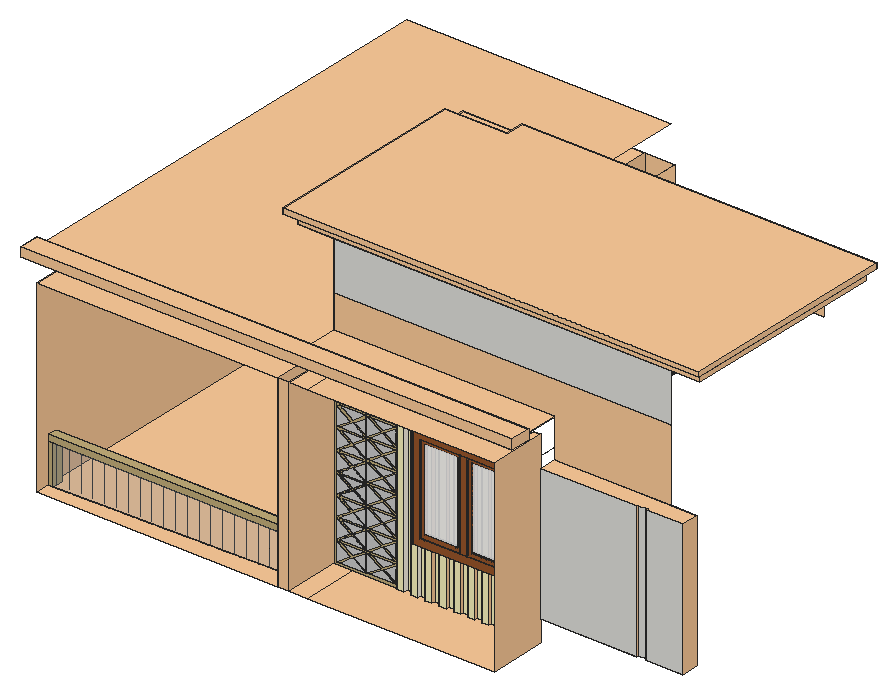
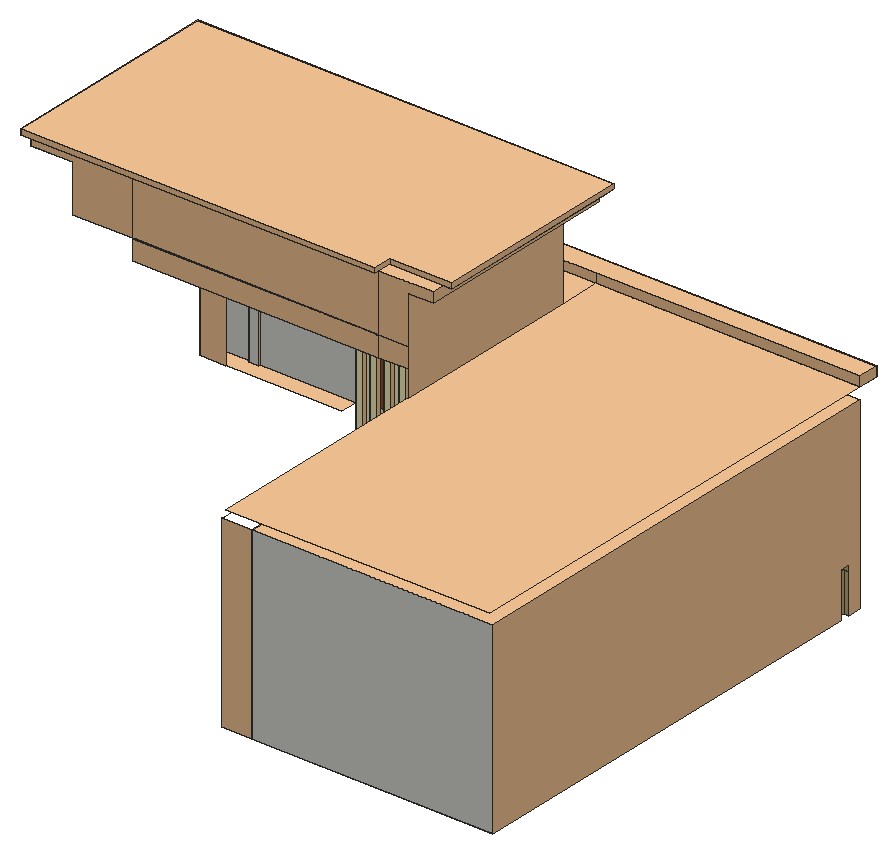
# SketchUp Ruby script. Lengths in inches.
U = 1.inch
M = Sketchup.active_model
def pt(a) = Geom::Point3d.new(a.map { |v| v * U })
def face(e, loops, mat)
  f = e.add_face(loops[0].map { |a| pt(a) })
  loops[1..].each { |l| e.add_face(l.map { |a| pt(a) }).erase! }
  f.material = f.back_material = mat if mat
  f
end
# faces: each face lists its corners as indices into pts; further lists are holes
def faces(e, pts, list, mat = nil) = list.each { |f| face(e, (f[0].is_a?(Array) ? f : [f]).map { |l| l.map { |i| pts[i] } }, mat) }
# xy, xz, yz: faces in a plane at the given z, y or x. An outline is a flat list of corners, or four numbers for a rectangle; further outlines are holes
def ring(l) = l.size == 4 ? [[l[0], l[1]], [l[2], l[1]], [l[2], l[3]], [l[0], l[3]]] : l.each_slice(2).to_a
def flat(e, list, mat, &to3) = list.each { |f| face(e, (f[0].is_a?(Array) ? f : [f]).map { |l| ring(l).map { |u, v| to3.(u, v) } }, mat) }
def xy(e, z, list, mat = nil) = flat(e, list, mat) { |x, y| [x, y, z] }
def xz(e, y, list, mat = nil) = flat(e, list, mat) { |x, z| [x, y, z] }
def yz(e, x, list, mat = nil) = flat(e, list, mat) { |y, z| [x, y, z] }
def lines(e, pts, list) = list.each { |a, b| e.add_line(pt(pts[a]), pt(pts[b])) }
# prism: a flat outline (further loops are holes) pulled along v
def prism(e, loops, v, mat = nil)
  f = face(e, loops, mat); d = Geom::Vector3d.new(v.map { |x| x * U })
  f.pushpull(f.normal.samedirection?(d) ? d.length : -d.length)
end
def box(e, o, s, mat = nil) = prism(e, [[o, [o[0] + s[0], o[1], o[2]], [o[0] + s[0], o[1] + s[1], o[2]], [o[0], o[1] + s[1], o[2]]]], [0, 0, s[2]], mat)
def at(x, y, z, deg = 0) = Geom::Transformation.translation(pt([x, y, z])) * Geom::Transformation.rotation(ORIGIN, Z_AXIS, deg.degrees)
def axes(o, x, y, z) = Geom::Transformation.new([*x, 0, *y, 0, *z, 0, *pt(o).to_a, 1])
def part(name) = M.definitions.add(name)
# library, detail: a bought-in or finely detailed component or shape, given as its bounding box
def library(name, o, s) = part(name).tap { |d| box(d.entities, o, s) }
def detail(e, o, s) = box(e.add_group.entities, o, s)
def put(e, d, t, mat = nil) = e.add_instance(d, t).tap { |i| i.material = mat if mat }
def group(e, t, mat = nil) = e.add_group.tap { |g| g.transformation = t; g.material = mat if mat }.entities
root = M.entities
M.materials.add("C02_Golden_Beige").color = [255, 205, 155]
M.materials.add("D02_Buttercup_Glow").color = [255, 248, 232]
M.materials.add("Glass_Basic_1").color = [161, 173, 186]
M.materials["Glass_Basic_1"].alpha = 0.25
M.materials.add("Metal_10_1K").color = [196, 175, 123]
M.materials.add("Metal_Perforated_03_1K").color = [205, 205, 205]
M.materials.add("Wood_Floor_01_1K").color = [255, 248, 193]
M.materials.add("[Translucent Glass Sky Reflection]").color = [253, 253, 253]
M.materials["[Translucent Glass Sky Reflection]"].alpha = 0.9
M.materials.add("[Wood Cherry Original]").color = [152, 86, 42]
c1 = library("Windows_Triple-Wood-Casement-Window-51inx36in",[0,0,-2.19],[51,41,3.19])
c2 = part("WINDOW")
g1 = group(c2.entities,at(4,1,4),"[Translucent Glass Sky Reflection]")
xy(g1,0,[[0,0,22,2]])
xy(g1,2,[[2,0,20,0.68],[2,0.68,20,2]],"[Wood Cherry Original]")
xy(g1,46,[[2,0,20,0.68],[2,0.68,20,2]],"[Wood Cherry Original]")
xy(g1,48,[[0,0,22,2]])
xz(g1,0,[[[0,0,22,48],[2,2,20,46]]],"[Wood Cherry Original]")
xz(g1,0.68,[[2,2,20,46]])
xz(g1,2,[[[0,0,22,48],[2,2,20,46]]],"[Wood Cherry Original]")
yz(g1,0,[[0,0,2,48]])
yz(g1,2,[[0,2,0.68,46],[0.68,2,2,46]],"[Wood Cherry Original]")
yz(g1,20,[[0,2,0.68,46],[0.68,2,2,46]],"[Wood Cherry Original]")
yz(g1,22,[[0,0,2,48]])
g2 = group(c2.entities,at(30,1,4),"[Translucent Glass Sky Reflection]")
xy(g2,0,[[0,0,22,2]])
xy(g2,2,[[2,0,20,0.68],[2,0.68,20,2]],"[Wood Cherry Original]")
xy(g2,46,[[2,0,20,0.68],[2,0.68,20,2]],"[Wood Cherry Original]")
xy(g2,48,[[0,0,22,2]])
xz(g2,0,[[[0,0,22,48],[2,2,20,46]]],"[Wood Cherry Original]")
xz(g2,0.68,[[2,2,20,46]])
xz(g2,2,[[[0,0,22,48],[2,2,20,46]]],"[Wood Cherry Original]")
yz(g2,0,[[0,0,2,48]])
yz(g2,2,[[0,2,0.68,46],[0.68,2,2,46]],"[Wood Cherry Original]")
yz(g2,20,[[0,2,0.68,46],[0.68,2,2,46]],"[Wood Cherry Original]")
yz(g2,22,[[0,0,2,48]])
g3 = group(c2.entities,at(0,0,0),"[Wood Cherry Original]")
xy(g3,0,[[0,0,56,4]])
xy(g3,4,[[4,0,26,4],[26,0,30,4],[30,0,52,4]])
xy(g3,52,[[4,0,26,4],[26,0,30,4],[30,0,52,4]])
xy(g3,56,[[0,0,56,4]])
xz(g3,0,[[[0,0,56,56],[4,4,52,52]],[26,4,30,52]])
xz(g3,4,[[[0,0,56,56],[4,4,52,52]],[26,4,30,52]])
yz(g3,0,[[0,0,4,56]])
yz(g3,4,[[0,4,4,52]])
yz(g3,26,[[0,4,4,52]])
yz(g3,30,[[0,4,4,52]])
yz(g3,52,[[0,4,4,52]])
yz(g3,56,[[0,0,4,56]])
xy(root,164.341,[[453.588,382.491,622.52,382.491,622.52,396.249,457.114,392.701,453.588,392.701],[630.52,382.491,643.626,422.102],[643.626,382.491,774.437,382.491,774.437,422.996,769.485,422.996,769.485,420.858,764.533,420.858,764.533,422.996,759.581,422.996,759.581,420.858,754.629,420.858,754.629,422.996,749.677,422.996,749.677,420.858,744.725,420.858,744.725,422.996,739.773,422.996,739.773,420.858,734.821,420.858,734.821,422.996,729.869,422.996,729.869,420.858,724.917,420.858,724.917,422.996,719.965,422.996,719.965,420.858,715.013,420.858,715.013,422.996,710.061,422.996,710.061,420.858,705.109,420.858,705.109,422.996,700.157,422.996,700.157,420.858,695.205,420.858,695.205,422.996,690.253,422.996,690.253,420.858,685.301,420.858,685.301,424.064,680.349,424.064,680.349,420.858,675.397,420.858,675.397,422.102,643.626,422.102],[457.114,392.701,622.52,396.249,622.52,703.99,453.588,703.99,453.588,399.796,457.114,399.796]],"C02_Golden_Beige")
xy(root,189.298,[[784.979,409.652,784.979,422.102,884.742,422.102,884.742,409.652,859.112,409.652,859.112,410.875,852.431,410.875,852.431,409.652]],"C02_Golden_Beige")
xy(root,191.701,[[457.114,392.701,457.114,399.796,622.52,399.796,622.52,396.249],[457.114,392.701,622.52,396.249,622.52,392.701]],"Metal_10_1K")
xy(root,196.087,[[453.588,392.701,622.52,399.796]],"Metal_10_1K")
xy(root,283.565,[[784.979,409.652,852.431,409.652,852.431,410.875,859.112,410.875,859.112,409.652,884.742,409.652,884.742,422.102,784.979,422.102]],"C02_Golden_Beige")
xy(root,295.512,[[[453.588,382.491,622.52,703.99],[484.212,419.811,491.847,605.683],[563.338,419.811,570.973,605.683]],[630.52,382.491,643.626,422.102],[643.626,382.491,643.626,422.102,675.397,422.102,675.397,420.858,680.349,420.858,680.349,424.064,685.301,424.064,685.301,420.858,690.253,420.858,690.253,422.996,695.205,422.996,695.205,420.858,700.157,420.858,700.157,422.996,705.109,422.996,705.109,420.858,710.061,420.858,710.061,422.996,715.013,422.996,715.013,420.858,719.965,420.858,719.965,422.996,724.917,422.996,724.917,420.858,729.869,420.858,729.869,422.996,734.821,422.996,734.821,420.858,739.773,420.858,739.773,422.996,744.725,422.996,744.725,420.858,749.677,420.858,749.677,422.996,754.629,422.996,754.629,420.858,759.581,420.858,759.581,422.996,764.533,422.996,764.533,420.858,769.485,420.858,769.485,422.996,774.437,422.996,774.437,382.491]],"C02_Golden_Beige")
xy(root,296.545,[[484.212,419.811,491.847,605.683]],"C02_Golden_Beige")
xy(root,298.092,[[563.338,419.811,570.973,605.683]],"C02_Golden_Beige")
xy(root,311.036,[[445.588,378.263,790.029,382.491],[445.588,382.491,784.979,392.701],[784.979,382.491,790.029,392.701],[445.588,392.701,630.52,716.631],[630.52,392.701,784.979,422.102]],"C02_Golden_Beige")
xy(root,317.496,[[445.588,378.263,790.029,392.701]],"C02_Golden_Beige")
xy(root,376.07,[[613.616,411.241,630.52,556.188],[630.52,411.241,895.57,422.102],[866.193,422.102,895.57,556.188]],"C02_Golden_Beige")
xy(root,383.319,[[608.019,405.157,899.824,411.241],[608.019,411.241,613.616,547.254],[895.57,411.241,899.824,560.283],[613.616,547.254,651.626,556.188],[651.626,556.188,823.98,560.283],
  [823.98,556.188,895.57,560.283]],"C02_Golden_Beige")
xy(root,386.847,[[608.019,405.157,899.824,405.157,899.824,560.283,651.626,560.283,651.626,547.254,608.019,547.254]],"C02_Golden_Beige")
xz(root,378.263,[[445.588,311.036,790.029,317.496]],"C02_Golden_Beige")
xz(root,382.491,[[622.52,164.341,630.52,295.512]],"C02_Golden_Beige")
xz(root,392.701,[[445.588,311.036,630.52,317.496],[630.52,311.036,790.029,317.496]],"C02_Golden_Beige")
xz(root,392.701,[[453.588,164.341,457.114,191.701],[453.588,191.701,622.52,196.087]],"Metal_10_1K")
xz(root,399.796,[[453.588,164.341,453.588,196.087,622.52,196.087,622.52,191.701,457.114,191.701,457.114,164.341]],"C02_Golden_Beige")
xz(root,405.157,[[608.019,383.319,899.824,386.847]],"C02_Golden_Beige")
xz(root,409.652,[[784.979,189.298,852.431,283.565],[859.112,189.298,884.742,283.565]])
xz(root,410.875,[[852.431,189.298,859.112,283.565]])
xz(root,411.241,[[613.616,376.07,895.57,383.319]],"C02_Golden_Beige")
xz(root,419.811,[[484.212,295.512,491.847,296.545],[563.338,295.512,570.973,298.092]],"C02_Golden_Beige")
xz(root,420.858,[[675.397,164.341,680.349,295.512],[685.301,164.341,690.253,295.512],[695.205,164.341,700.157,295.512],[705.109,164.341,710.061,295.512],[715.013,164.341,719.965,295.512],
  [724.917,164.341,729.869,295.512],[734.821,164.341,739.773,295.512],[744.725,164.341,749.677,295.512],[754.629,164.341,759.581,295.512],[764.533,164.341,769.485,295.512]],"Wood_Floor_01_1K")
xz(root,422.102,[[652.387,166.24,652.391,179.253],[652.387,180.373,652.387,180.535,652.139,180.535],[652.387,265.24,652.391,266.349],[652.387,266.349,652.391,279.363],[632.419,279.363,652.387,279.49],
  [630.52,334.01,866.193,376.07]])
xz(root,422.102,[[866.193,189.298,884.742,283.565],[784.979,283.565,866.193,283.565,866.193,334.01,630.52,334.01,630.52,311.036,784.979,311.036]],"C02_Golden_Beige")
xz(root,422.102,[[[630.52,164.341,675.397,295.512],[632.419,166.24,673.498,293.613]],[632.419,166.24,634.334,166.24,643.309,172.156,652.387,166.24,652.387,167.401,644.224,172.76,652.387,178.14,652.387,179.253,643.327,173.349,634.334,179.253,632.419,179.253,642.403,172.747],[[632.419,166.24,634.334,166.24,643.309,172.156,652.387,166.24,652.387,167.401,644.224,172.76,652.387,178.14,652.387,181.534,644.224,186.893,652.387,192.274,652.387,195.667,644.224,201.026,652.387,206.407,652.387,209.8,644.224,215.159,652.387,220.54,652.387,223.934,644.224,229.293,652.387,234.673,652.387,238.067,644.224,243.426,652.387,248.807,652.387,251.201,652.139,251.201,652.387,251.039,632.419,251.039,632.419,249.92,642.403,243.413,632.419,236.906,634.334,236.906,634.579,237.068,643.309,242.822,652.387,236.906,632.419,236.906,632.419,235.786,642.403,229.279,632.419,222.773,634.334,222.773,643.309,228.689,652.387,222.773,632.419,222.773,632.419,221.653,642.403,215.146,632.419,208.639,634.334,208.639,643.309,214.556,652.387,208.639,632.419,208.639,632.419,207.52,642.403,201.013,632.419,194.506,634.334,194.506,643.309,200.423,652.387,194.506,632.419,194.506,632.419,193.387,642.403,186.88,632.419,180.373,634.334,180.373,643.309,186.289,652.139,180.535,652.387,180.373,632.419,180.373,632.419,179.253,642.403,172.747],[643.327,173.349,634.334,179.253,652.387,179.253],[643.327,187.482,634.334,193.387,652.387,193.387],[643.327,201.615,634.334,207.52,652.387,207.52],[643.327,215.749,634.334,221.653,652.387,221.653],[643.327,229.882,634.334,235.786,652.387,235.786],[643.327,244.015,634.334,249.92,652.387,249.92]],[652.391,166.24,653.525,166.24,653.525,279.49,652.387,279.49,652.387,279.363,652.391,279.363,652.391,265.24,652.387,265.24,652.387,179.253,652.391,179.253],[653.525,166.24,655.44,166.24,664.415,172.156,673.493,166.24,673.493,167.401,665.331,172.76,673.493,178.14,673.493,179.253,664.434,173.349,655.44,179.253,653.525,179.253,663.509,172.747],
  [653.525,179.253,673.498,180.535],[632.419,180.373,634.334,180.373,643.309,186.289,652.139,180.535,652.387,180.535,652.387,181.534,644.224,186.893,652.387,192.274,652.387,193.387,643.327,187.482,634.334,193.387,632.419,193.387,642.403,186.88],[653.525,180.535,655.44,180.535,664.415,186.451,673.493,180.535,673.493,181.696,665.331,187.055,673.493,192.435,673.493,193.548,664.434,187.644,655.44,193.548,653.525,193.548,663.509,187.042],[653.525,193.548,673.498,194.83],[632.419,194.506,634.334,194.506,643.309,200.423,652.387,194.506,652.387,195.667,644.224,201.026,652.387,206.407,652.387,207.52,643.327,201.615,634.334,207.52,632.419,207.52,642.403,201.013],
  [653.525,194.83,655.44,194.83,664.415,200.746,673.493,194.83,673.493,195.991,665.331,201.35,673.493,206.73,673.493,207.843,664.434,201.939,655.44,207.843,653.525,207.843,663.509,201.336],[653.525,207.843,673.498,209.125],[632.419,208.639,634.334,208.639,643.309,214.556,652.387,208.639,652.387,209.8,644.224,215.159,652.387,220.54,652.387,221.653,643.327,215.749,634.334,221.653,632.419,221.653,642.403,215.146],[653.525,209.125,655.44,209.125,664.415,215.041,673.493,209.125,673.493,210.285,665.331,215.644,673.493,221.025,673.493,222.138,664.434,216.234,655.44,222.138,653.525,222.138,663.509,215.631],[653.525,222.138,673.498,223.419],
  [632.419,222.773,634.334,222.773,643.309,228.689,652.387,222.773,652.387,223.934,644.224,229.293,652.387,234.673,652.387,235.786,643.327,229.882,634.334,235.786,632.419,235.786,642.403,229.279],[653.525,223.419,655.44,223.419,664.415,229.336,673.493,223.419,673.493,224.58,665.331,229.939,673.493,235.32,673.493,236.433,664.434,230.529,655.44,236.433,653.525,236.433,663.509,229.926],[653.525,236.433,673.498,237.714],[632.419,236.906,634.334,236.906,634.579,237.068,643.309,242.822,652.387,236.906,652.387,238.067,644.224,243.426,652.387,248.807,652.387,249.92,643.327,244.015,634.334,249.92,632.419,249.92,642.403,243.413],[653.525,237.714,655.44,237.714,664.415,243.631,673.493,237.714,673.493,238.875,665.331,244.234,673.493,249.615,673.493,250.728,664.434,244.823,655.44,250.728,653.525,250.728,663.509,244.221],
  [653.525,250.728,673.498,252.009],[632.419,251.039,634.334,251.039,643.309,256.955,652.139,251.201,652.387,251.201,652.387,252.2,644.224,257.559,652.387,262.94,652.387,265.392,643.327,258.148,634.334,265.392,632.419,264.053,642.403,257.546],[653.525,252.009,655.44,252.009,664.415,257.926,673.493,252.009,673.493,253.17,665.331,258.529,673.493,263.91,673.493,265.023,664.434,259.118,655.44,265.023,653.525,265.023,663.509,258.516],[632.419,264.053,634.334,265.392,652.387,265.392,652.387,267.51,644.224,272.869,652.387,278.25,652.387,279.363,643.327,273.458,634.334,279.363,632.419,279.363,642.403,272.856,632.419,266.349,634.334,266.349,643.309,272.265,652.387,266.349,632.419,266.349],[653.525,265.023,673.498,266.304],
  [653.525,266.304,655.44,266.304,664.415,272.221,673.493,266.304,673.493,267.465,665.331,272.824,673.493,278.205,673.493,279.318,664.434,273.413,655.44,279.318,653.525,279.318,663.509,272.811],[632.419,279.49,652.387,280.599],[652.387,279.49,653.525,280.599],[653.525,279.49,673.498,280.599],[632.419,280.599,634.334,280.599,643.309,286.516,652.387,280.599,652.387,281.76,644.224,287.119,652.387,292.5,652.387,293.613,643.327,287.708,634.334,293.613,632.419,293.613,642.403,287.106],
  [652.387,280.599,653.525,293.613],[653.525,280.599,655.44,280.599,664.415,286.516,673.493,280.599,673.493,281.76,665.331,287.119,673.493,292.5,673.493,293.613,664.434,287.708,655.44,293.613,653.525,293.613,663.509,287.106]],"Metal_10_1K")
xz(root,422.102,[[632.419,166.24,642.403,172.747,632.419,179.253],[634.334,166.24,652.387,166.24,643.309,172.156],[653.525,166.24,663.509,172.747,653.525,179.253],[655.44,166.24,673.493,166.24,664.415,172.156],[673.493,166.24,673.498,166.24,673.498,179.253,673.493,179.253,673.493,178.14,665.331,172.76,673.493,167.401],
  [652.387,167.401,652.387,178.14,644.224,172.76],[643.327,173.349,652.387,179.253,634.334,179.253],[664.434,173.349,673.493,179.253,655.44,179.253],[632.419,180.373,642.403,186.88,632.419,193.387],[634.334,180.373,652.387,180.373,652.139,180.535,643.309,186.289],
  [653.525,180.535,663.509,187.042,653.525,193.548],[655.44,180.535,673.493,180.535,664.415,186.451],[673.493,180.535,673.498,180.535,673.498,193.548,673.493,193.548,673.493,192.435,665.331,187.055,673.493,181.696],[652.387,181.534,652.387,192.274,644.224,186.893],[643.327,187.482,652.387,193.387,634.334,193.387],
  [664.434,187.644,673.493,193.548,655.44,193.548],[632.419,194.506,642.403,201.013,632.419,207.52],[634.334,194.506,652.387,194.506,643.309,200.423],[653.525,194.83,663.509,201.336,653.525,207.843],[655.44,194.83,673.493,194.83,664.415,200.746],
  [673.493,194.83,673.498,194.83,673.498,207.843,673.493,207.843,673.493,206.73,665.331,201.35,673.493,195.991],[652.387,195.667,652.387,206.407,644.224,201.026],[643.327,201.615,652.387,207.52,634.334,207.52],[664.434,201.939,673.493,207.843,655.44,207.843],[632.419,208.639,642.403,215.146,632.419,221.653],
  [634.334,208.639,652.387,208.639,643.309,214.556],[653.525,209.125,663.509,215.631,653.525,222.138],[655.44,209.125,673.493,209.125,664.415,215.041],[673.493,209.125,673.498,209.125,673.498,222.138,673.493,222.138,673.493,221.025,665.331,215.644,673.493,210.285],[652.387,209.8,652.387,220.54,644.224,215.159],
  [643.327,215.749,652.387,221.653,634.334,221.653],[664.434,216.234,673.493,222.138,655.44,222.138],[632.419,222.773,642.403,229.279,632.419,235.786],[634.334,222.773,652.387,222.773,643.309,228.689],[653.525,223.419,663.509,229.926,653.525,236.433],
  [655.44,223.419,673.493,223.419,664.415,229.336],[673.493,223.419,673.498,223.419,673.498,236.433,673.493,236.433,673.493,235.32,665.331,229.939,673.493,224.58],[652.387,223.934,652.387,234.673,644.224,229.293],[643.327,229.882,652.387,235.786,634.334,235.786],[664.434,230.529,673.493,236.433,655.44,236.433],
  [632.419,236.906,642.403,243.413,632.419,249.92],[634.334,236.906,652.387,236.906,643.309,242.822,634.579,237.068],[653.525,237.714,663.509,244.221,653.525,250.728],[655.44,237.714,673.493,237.714,664.415,243.631],[673.493,237.714,673.498,237.714,673.498,250.728,673.493,250.728,673.493,249.615,665.331,244.234,673.493,238.875],
  [652.387,238.067,652.387,248.807,644.224,243.426],[643.327,244.015,652.387,249.92,634.334,249.92],[664.434,244.823,673.493,250.728,655.44,250.728],[632.419,251.039,642.403,257.546,632.419,264.053],[634.334,251.039,652.387,251.039,652.139,251.201,643.309,256.955],
  [653.525,252.009,663.509,258.516,653.525,265.023],[655.44,252.009,673.493,252.009,664.415,257.926],[673.493,252.009,673.498,252.009,673.498,265.023,673.493,265.023,673.493,263.91,665.331,258.529,673.493,253.17],[652.387,252.2,652.387,262.94,644.224,257.559],[643.327,258.148,652.387,265.392,634.334,265.392],
  [664.434,259.118,673.493,265.023,655.44,265.023],[653.525,266.304,663.509,272.811,653.525,279.318],[655.44,266.304,673.493,266.304,664.415,272.221],[673.493,266.304,673.498,266.304,673.498,279.318,673.493,279.318,673.493,278.205,665.331,272.824,673.493,267.465],[632.419,266.349,642.403,272.856,632.419,279.363],
  [634.334,266.349,652.387,266.349,643.309,272.265],[652.387,267.51,652.387,278.25,644.224,272.869],[664.434,273.413,673.493,279.318,673.498,279.318,673.498,279.49,653.525,279.49,653.525,279.318,655.44,279.318],[643.327,273.458,652.387,279.363,634.334,279.363],[632.419,280.599,642.403,287.106,632.419,293.613],
  [634.334,280.599,652.387,280.599,643.309,286.516],[653.525,280.599,663.509,287.106,653.525,293.613],[655.44,280.599,673.493,280.599,664.415,286.516],[673.493,280.599,673.498,280.599,673.498,293.613,673.493,293.613,673.493,292.5,665.331,287.119,673.493,281.76],[652.387,281.76,652.387,292.5,644.224,287.119],
  [643.327,287.708,652.387,293.613,634.334,293.613],[664.434,287.708,673.493,293.613,655.44,293.613]],"Metal_Perforated_03_1K")
xz(root,422.996,[[690.253,164.341,695.205,295.512],[700.157,164.341,705.109,295.512],[710.061,164.341,715.013,295.512],[719.965,164.341,724.917,295.512],[729.869,164.341,734.821,295.512],
  [739.773,164.341,744.725,295.512],[749.677,164.341,754.629,295.512],[759.581,164.341,764.533,295.512],[769.485,164.341,774.437,295.512]],"Wood_Floor_01_1K")
xz(root,424.064,[[680.349,164.341,685.301,295.512]],"Wood_Floor_01_1K")
xz(root,547.254,[[608.019,383.319,651.626,386.847]],"C02_Golden_Beige")
xz(root,556.188,[[630.52,328.718,651.626,342.851],[651.626,328.718,823.98,342.851],[630.52,342.851,630.52,376.07,613.616,376.07,613.616,383.319,651.626,383.319,651.626,342.851],[651.626,342.851,823.98,342.968],[651.626,342.968,823.98,383.319],
  [823.98,342.968,823.98,383.319,895.57,383.319,895.57,376.07,866.193,376.07,866.193,342.968]],"C02_Golden_Beige")
xz(root,560.283,[[651.626,383.319,899.824,386.847]],"C02_Golden_Beige")
xz(root,605.683,[[484.212,295.512,491.847,296.545],[563.338,295.512,570.973,298.092]],"C02_Golden_Beige")
xz(root,703.99,[[453.588,164.341,622.52,295.512]])
xz(root,703.99,[[622.52,164.341,643.626,295.512]],"C02_Golden_Beige")
yz(root,445.588,[[378.263,311.036,392.701,317.496]],"C02_Golden_Beige")
yz(root,453.588,[[382.491,164.341,392.701,164.341,392.701,196.087,399.796,196.087,399.796,164.341,703.99,164.341,703.99,295.512,382.491,295.512]],"C02_Golden_Beige")
yz(root,457.114,[[392.701,164.341,396.249,191.701],[396.249,164.341,399.796,191.701]],"Metal_10_1K")
yz(root,484.212,[[419.811,295.512,605.683,296.545]],"C02_Golden_Beige")
yz(root,491.847,[[419.811,295.512,605.683,296.545]],"C02_Golden_Beige")
yz(root,563.338,[[419.811,295.512,605.683,298.092]],"C02_Golden_Beige")
yz(root,570.973,[[419.811,295.512,605.683,298.092]],"C02_Golden_Beige")
yz(root,608.019,[[405.157,383.319,547.254,386.847]],"C02_Golden_Beige")
yz(root,613.616,[[411.241,376.07,556.188,383.319]],"C02_Golden_Beige")
yz(root,622.52,[[382.491,164.341,382.491,295.512,703.99,295.512,703.99,164.341,396.249,164.341,396.249,191.701,399.796,191.701,399.796,196.087,392.701,196.087,392.701,191.701,396.249,191.701,396.249,164.341]],"C02_Golden_Beige")
yz(root,630.52,[[382.491,164.341,422.102,295.512],[422.102,311.036,556.188,376.07]],"C02_Golden_Beige")
yz(root,651.626,[[547.254,383.319,560.283,386.847]],"C02_Golden_Beige")
yz(root,675.397,[[420.858,164.341,422.102,295.512]],"C02_Golden_Beige")
yz(root,680.349,[[420.858,164.341,424.064,295.512]],"D02_Buttercup_Glow")
yz(root,685.301,[[420.858,164.341,424.064,295.512]],"D02_Buttercup_Glow")
yz(root,690.253,[[420.858,164.341,422.996,295.512]],"D02_Buttercup_Glow")
yz(root,695.205,[[420.858,164.341,422.996,295.512]],"D02_Buttercup_Glow")
yz(root,700.157,[[420.858,164.341,422.996,295.512]],"C02_Golden_Beige")
yz(root,705.109,[[420.858,164.341,422.996,295.512]],"C02_Golden_Beige")
yz(root,710.061,[[420.858,164.341,422.996,295.512]],"C02_Golden_Beige")
yz(root,715.013,[[420.858,164.341,422.996,295.512]],"C02_Golden_Beige")
yz(root,719.965,[[420.858,164.341,422.996,295.512]],"C02_Golden_Beige")
yz(root,724.917,[[420.858,164.341,422.996,295.512]],"C02_Golden_Beige")
yz(root,729.869,[[420.858,164.341,422.996,295.512]],"C02_Golden_Beige")
yz(root,734.821,[[420.858,164.341,422.996,295.512]],"C02_Golden_Beige")
yz(root,739.773,[[420.858,164.341,422.996,295.512]],"C02_Golden_Beige")
yz(root,744.725,[[420.858,164.341,422.996,295.512]],"C02_Golden_Beige")
yz(root,749.677,[[420.858,164.341,422.996,295.512]],"C02_Golden_Beige")
yz(root,754.629,[[420.858,164.341,422.996,295.512]],"C02_Golden_Beige")
yz(root,759.581,[[420.858,164.341,422.996,295.512]],"C02_Golden_Beige")
yz(root,764.533,[[420.858,164.341,422.996,295.512]],"C02_Golden_Beige")
yz(root,769.485,[[420.858,164.341,422.996,295.512]],"C02_Golden_Beige")
yz(root,774.437,[[382.491,164.341,422.996,295.512]],"C02_Golden_Beige")
yz(root,790.029,[[378.263,311.036,392.701,317.496]],"C02_Golden_Beige")
yz(root,852.431,[[409.652,189.298,410.875,283.565]],"C02_Golden_Beige")
yz(root,859.112,[[409.652,189.298,410.875,283.565]],"C02_Golden_Beige")
yz(root,884.742,[[409.652,189.298,422.102,283.565]],"C02_Golden_Beige")
yz(root,895.57,[[411.241,376.07,556.188,383.319]],"C02_Golden_Beige")
yz(root,899.824,[[405.157,383.319,560.283,386.847]],"C02_Golden_Beige")
p = [[457.114,392.701,164.341],[622.52,396.249,164.341],[622.52,396.249,191.701],[457.114,392.701,191.701],[643.626,422.102,164.341],[643.626,703.99,164.341],
  [643.626,422.102,295.512],[643.626,703.99,295.512],[652.391,422.102,193.387],[652.387,422.102,193.387],[652.391,422.102,180.373],[652.391,422.102,207.52],
  [652.387,422.102,207.52],[652.391,422.102,194.506],[652.391,422.102,221.653],[652.387,422.102,221.653],[652.391,422.102,208.639],[652.391,422.102,235.786],
  [652.387,422.102,235.786],[652.391,422.102,222.773],[634.334,422.102,237.068],[634.579,422.102,237.068],[652.391,422.102,249.92],[652.387,422.102,249.92],
  [652.391,422.102,236.906],[652.391,422.102,264.053],[652.387,422.102,265.24],[652.391,422.102,251.039],[465.384,396.249,164.341],[465.384,396.249,191.701],
  [473.654,396.249,164.341],[473.654,396.249,191.701],[481.924,396.249,164.341],[481.924,396.249,191.701],[490.195,396.249,164.341],[490.195,396.249,191.701],
  [498.465,396.249,164.341],[498.465,396.249,191.701],[506.735,396.249,164.341],[506.735,396.249,191.701],[515.006,396.249,164.341],[515.006,396.249,191.701],
  [523.276,396.249,164.341],[523.276,396.249,191.701],[531.546,396.249,164.341],[531.546,396.249,191.701],[539.817,396.249,164.341],[539.817,396.249,191.701],
  [548.087,396.249,164.341],[548.087,396.249,191.701],[556.357,396.249,164.341],[556.357,396.249,191.701],[564.628,396.249,164.341],[564.628,396.249,191.701],
  [572.898,396.249,164.341],[572.898,396.249,191.701],[581.168,396.249,164.341],[581.168,396.249,191.701],[589.438,396.249,164.341],[589.438,396.249,191.701],
  [597.709,396.249,164.341],[597.709,396.249,191.701],[605.979,396.249,164.341],[605.979,396.249,191.701],[614.249,396.249,164.341],[614.249,396.249,191.701]]
faces(root,p,[[0,1,2,3]],"Glass_Basic_1")
lines(root,p,[[4,5],[6,7],[8,9],[10,8],[11,12],[13,11],[14,15],[16,14],[17,18],[19,17],[20,21],[22,23],
  [24,22],[25,26],[27,25],[28,29],[30,31],[32,33],[34,35],[36,37],[38,39],[40,41],[42,43],[44,45],
  [46,47],[48,49],[50,51],[52,53],[54,55],[56,57],[58,59],[60,61],[62,63],[64,65]])
put(root,c1,axes([486.04,699.37,182.58],[1.67137,0,0],[0,0,1.86328],[0,-1,0]))
put(root,c2,axes([689.43,416.86,199.54],[1.28,0,0],[0,1,0],[0,0,1.3]))
